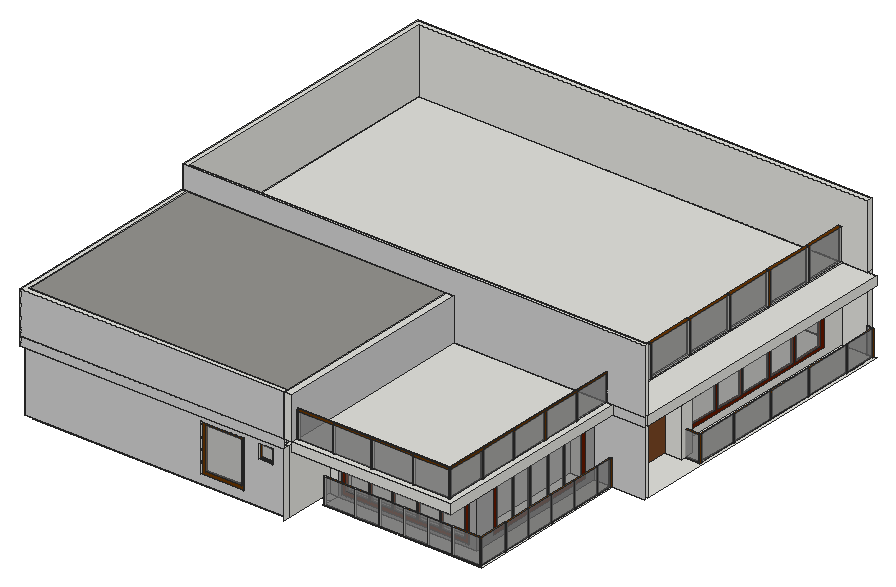
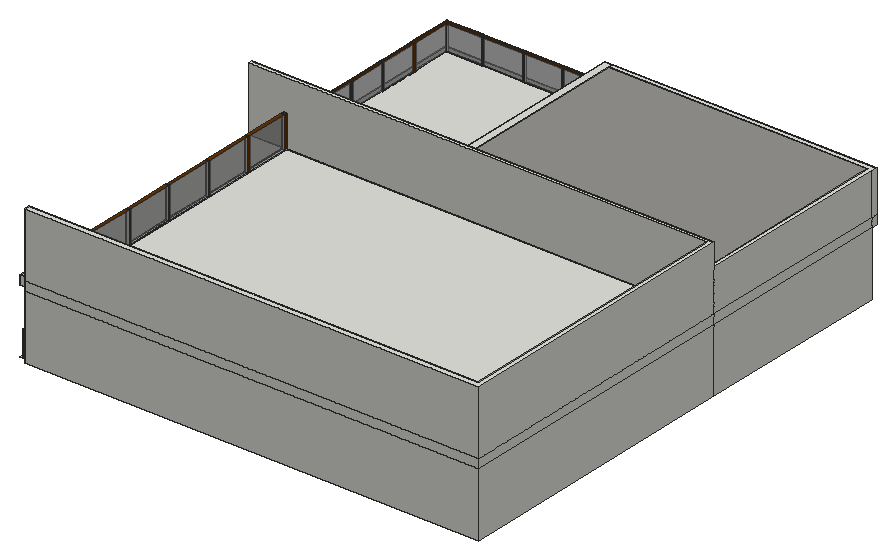
# SketchUp Ruby script. Lengths in inches.
U = 1.inch
M = Sketchup.active_model
def pt(a) = Geom::Point3d.new(a.map { |v| v * U })
def face(e, loops, mat)
  f = e.add_face(loops[0].map { |a| pt(a) })
  loops[1..].each { |l| e.add_face(l.map { |a| pt(a) }).erase! }
  f.material = f.back_material = mat if mat
  f
end
# faces: each face lists its corners as indices into pts; further lists are holes
def faces(e, pts, list, mat = nil) = list.each { |f| face(e, (f[0].is_a?(Array) ? f : [f]).map { |l| l.map { |i| pts[i] } }, mat) }
# xy, xz, yz: faces in a plane at the given z, y or x. An outline is a flat list of corners, or four numbers for a rectangle; further outlines are holes
def ring(l) = l.size == 4 ? [[l[0], l[1]], [l[2], l[1]], [l[2], l[3]], [l[0], l[3]]] : l.each_slice(2).to_a
def flat(e, list, mat, &to3) = list.each { |f| face(e, (f[0].is_a?(Array) ? f : [f]).map { |l| ring(l).map { |u, v| to3.(u, v) } }, mat) }
def xy(e, z, list, mat = nil) = flat(e, list, mat) { |x, y| [x, y, z] }
def xz(e, y, list, mat = nil) = flat(e, list, mat) { |x, z| [x, y, z] }
def yz(e, x, list, mat = nil) = flat(e, list, mat) { |y, z| [x, y, z] }
def lines(e, pts, list) = list.each { |a, b| e.add_line(pt(pts[a]), pt(pts[b])) }
# prism: a flat outline (further loops are holes) pulled along v
def prism(e, loops, v, mat = nil)
  f = face(e, loops, mat); d = Geom::Vector3d.new(v.map { |x| x * U })
  f.pushpull(f.normal.samedirection?(d) ? d.length : -d.length)
end
def box(e, o, s, mat = nil) = prism(e, [[o, [o[0] + s[0], o[1], o[2]], [o[0] + s[0], o[1] + s[1], o[2]], [o[0], o[1] + s[1], o[2]]]], [0, 0, s[2]], mat)
def at(x, y, z, deg = 0) = Geom::Transformation.translation(pt([x, y, z])) * Geom::Transformation.rotation(ORIGIN, Z_AXIS, deg.degrees)
def axes(o, x, y, z) = Geom::Transformation.new([*x, 0, *y, 0, *z, 0, *pt(o).to_a, 1])
def part(name) = M.definitions.add(name)
# library, detail: a bought-in or finely detailed component or shape, given as its bounding box
def library(name, o, s) = part(name).tap { |d| box(d.entities, o, s) }
def detail(e, o, s) = box(e.add_group.entities, o, s)
def put(e, d, t, mat = nil) = e.add_instance(d, t).tap { |i| i.material = mat if mat }
def group(e, t, mat = nil) = e.add_group.tap { |g| g.transformation = t; g.material = mat if mat }.entities
root = M.entities
M.materials.add("[Carrera Marble]").color = [207, 207, 207]
M.materials.add("[Color B08]").color = [102, 25, 0]
M.materials.add("[Color C08]").color = [102, 51, 0]
M.materials.add("[Granite Light Gray]").color = [149, 148, 144]
M.materials.add("[Stone Vein Gray]").color = [166, 165, 165]
M.materials.add("[Translucent Glass Gray]").color = [128, 128, 128]
M.materials["[Translucent Glass Gray]"].alpha = 0.5
M.materials.add("[Wood Veneer 01]").color = [120, 70, 37]
c1 = part("Group\#3")
xy(c1.entities,0,[[0,0,23.0625,440.625]],"[Color B08]")
xy(c1.entities,14.28,[[0,14.28,23.0625,92.65],[0,98.4,23.0625,173.71],[0,179.46,23.0625,261.65],[0,267.4,23.0625,340.59],[0,346.34,23.0625,426.35]],"[Color B08]")
xy(c1.entities,204.03,[[0,14.28,23.0625,92.65],[0,98.4,23.0625,173.71],[0,179.46,23.0625,261.65],[0,267.4,23.0625,340.59],[0,346.34,23.0625,426.35]],"[Color B08]")
xy(c1.entities,218.3125,[[0,0,23.0625,440.625]],"[Color B08]")
xz(c1.entities,0,[[0,0,23.0625,218.3125]],"[Color B08]")
xz(c1.entities,14.28,[[0,14.28,23.0625,204.03]],"[Color B08]")
xz(c1.entities,92.65,[[0,14.28,23.0625,204.03]],"[Color B08]")
xz(c1.entities,98.4,[[0,14.28,23.0625,204.03]],"[Color B08]")
xz(c1.entities,173.71,[[0,14.28,23.0625,204.03]],"[Color B08]")
xz(c1.entities,179.46,[[0,14.28,23.0625,204.03]],"[Color B08]")
xz(c1.entities,261.65,[[0,14.28,23.0625,204.03]],"[Color B08]")
xz(c1.entities,267.4,[[0,14.28,23.0625,204.03]],"[Color B08]")
xz(c1.entities,340.59,[[0,14.28,23.0625,204.03]],"[Color B08]")
xz(c1.entities,346.34,[[0,14.28,23.0625,204.03]],"[Color B08]")
xz(c1.entities,426.35,[[0,14.28,23.0625,204.03]],"[Color B08]")
xz(c1.entities,440.625,[[0,0,23.0625,218.3125]],"[Color B08]")
yz(c1.entities,0,[[[0,0,440.625,218.3125],[179.46,14.28,261.65,204.03],[346.34,14.28,426.35,204.03],[14.28,14.28,92.65,204.03],[98.4,14.28,173.71,204.03],[267.4,14.28,340.59,204.03]]],"[Color B08]")
yz(c1.entities,23.0625,[[[0,0,440.625,218.3125],[179.46,14.28,261.65,204.03],[346.34,14.28,426.35,204.03],[14.28,14.28,92.65,204.03],[98.4,14.28,173.71,204.03],[267.4,14.28,340.59,204.03]]],"[Color B08]")
yz(c1.entities,23.0625,[[14.28,14.28,92.65,204.03],[98.4,14.28,173.71,204.03],[179.46,14.28,261.65,204.03],[267.4,14.28,340.59,204.03],[346.34,14.28,426.35,204.03]],"[Translucent Glass Gray]")
c2 = part("Group\#1")
xy(c2.entities,0,[[0,0,21.625,260.4375]],"[Color C08]")
xy(c2.entities,20.42,[[0,20.42,21.625,240.02]],"[Color C08]")
xy(c2.entities,312.95,[[0,20.42,21.625,240.02]],"[Color C08]")
xy(c2.entities,333.375,[[0,0,21.625,260.4375]],"[Color C08]")
xz(c2.entities,0,[[0,0,21.625,333.375]],"[Color C08]")
xz(c2.entities,20.42,[[0,20.42,21.625,312.95]],"[Color C08]")
xz(c2.entities,240.02,[[0,20.42,21.625,312.95]],"[Color C08]")
xz(c2.entities,260.4375,[[0,0,21.625,333.375]],"[Color C08]")
yz(c2.entities,0,[[[0,0,260.4375,333.375],[20.42,20.42,240.02,312.95]]],"[Color C08]")
yz(c2.entities,21.625,[[[0,0,260.4375,333.375],[20.42,20.42,240.02,312.95]]],"[Color C08]")
yz(c2.entities,21.625,[[20.42,20.42,240.02,312.95]],"[Translucent Glass Gray]")
xy(root,960,[[9,213.0625,482.6875,573],[9,579,791.375,1111.6875]])
xy(root,966,[[0,207.0625,0,573,9,573,9,213.0625,482.6875,213.0625,482.6875,308.3125,607.75,308.3125,607.75,573,766.0625,573,766.0625,301.1875,491.3125,301.1875,491.3125,207.0625],[9,213.0625,482.6875,573],[506.0625,267.5625,801.71,267.5625,801.71,573,799.5,573,799.5,268.8125,506.0625,268.8125],[506.0625,268.8125,509.36,270.8125],[509.36,268.8125,564.18,270.8125],
  [564.18,268.8125,565.36,270.8125],[565.36,268.8125,609.49,270.8125],[609.49,268.8125,610.67,270.8125],[610.67,268.8125,654.81,270.8125],[654.81,268.8125,655.98,270.8125],
  [655.98,268.8125,700.12,270.8125],[700.12,268.8125,701.3,270.8125],[701.3,268.8125,745.43,270.8125],[745.43,268.8125,746.61,270.8125],[746.61,268.8125,797.5,270.8125],
  [797.5,268.8125,799.5,270.8125],[506.0625,270.8125,797.5,270.8125,797.5,573,766.0625,573,766.0625,301.1875,506.0625,301.1875],[797.5,270.8125,799.5,326.79],[491.3125,282.8125,506.0625,301.1875],[482.6875,308.3125,607.75,573],
  [797.5,326.79,799.5,327.91],[797.5,327.91,799.5,380.04],[797.5,380.04,799.5,381.16],[797.5,381.16,799.5,433.29],[797.5,433.29,799.5,434.41],
  [797.5,434.41,799.5,486.54],[797.5,486.54,799.5,487.66],[797.5,487.66,799.5,539.79],[797.5,539.79,799.5,540.91],[797.5,540.91,799.5,569.88],
  [797.5,569.88,799.5,573],[9,579,791.375,1111.6875],[797.375,579,861.375,579,861.375,1111.6875,797.375,1111.6875,797.375,723.02,828.5625,723.02,828.5625,710.0625,854.8125,710.0625,854.8125,1110.1875,845.0625,1110.1875,845.0625,1110.75,856.8125,1110.75,856.8125,706.6875,828.5625,706.6875,828.5625,699.0625,797.375,699.0625],[828.5625,706.6875,854.8125,710.0625],[854.8125,706.6875,856.8125,710.0625],
  [854.8125,710.0625,856.8125,784.92],[854.8125,784.92,856.8125,787.22],[854.8125,787.22,856.8125,872.67],[854.8125,872.67,856.8125,874.97],[854.8125,874.97,856.8125,960.42],
  [854.8125,960.42,856.8125,962.72],[854.8125,962.72,856.8125,1048.17],[854.8125,1048.17,856.8125,1050.47],[854.8125,1050.47,856.8125,1110.1875],[845.0625,1110.1875,854.8125,1110.75],
  [854.8125,1110.1875,856.8125,1110.75]])
xy(root,971.4,[[514.9,301.1875,750.72,321.75]])
xy(root,976.89,[[739.4375,339.98,766.0625,551.41]])
xy(root,976.93,[[791.375,750.16,797.375,1072.78]])
xy(root,981.52,[[327.22,207.0625,407.72,213.0625]])
xy(root,1014,[[506.0625,268.8125,509.36,270.8125],[509.36,268.8125,564.18,270.8125],[564.18,268.8125,565.36,270.8125],[565.36,268.8125,609.49,270.8125],[609.49,268.8125,610.67,270.8125],
  [610.67,268.8125,654.81,270.8125],[654.81,268.8125,655.98,270.8125],[655.98,268.8125,700.12,270.8125],[700.12,268.8125,701.3,270.8125],[701.3,268.8125,745.43,270.8125],
  [745.43,268.8125,746.61,270.8125],[746.61,268.8125,797.5,270.8125],[797.5,268.8125,799.5,270.8125],[797.5,270.8125,799.5,326.79],[797.5,326.79,799.5,327.91],
  [797.5,327.91,799.5,380.04],[797.5,380.04,799.5,381.16],[797.5,381.16,799.5,433.29],[797.5,433.29,799.5,434.41],[797.5,434.41,799.5,486.54],
  [797.5,486.54,799.5,487.66],[797.5,487.66,799.5,539.79],[797.5,539.79,799.5,540.91],[797.5,540.91,799.5,569.88],[797.5,569.88,799.5,573],
  [828.5625,706.6875,854.8125,710.0625],[854.8125,706.6875,856.8125,710.0625],[854.8125,710.0625,856.8125,784.92],[854.8125,784.92,856.8125,787.22],[854.8125,787.22,856.8125,872.67],
  [854.8125,872.67,856.8125,874.97],[854.8125,874.97,856.8125,960.42],[854.8125,960.42,856.8125,962.72],[854.8125,962.72,856.8125,1048.17],[854.8125,1048.17,856.8125,1050.47],
  [854.8125,1050.47,856.8125,1110.1875],[845.0625,1110.1875,854.8125,1110.75],[854.8125,1110.1875,856.8125,1110.75]],"[Color C08]")
xy(root,1044.6875,[[434.39,207.0625,461.57,213.0625]])
xy(root,1070.65,[[327.22,207.0625,407.72,213.0625]])
xy(root,1071.875,[[434.39,207.0625,461.57,213.0625]])
xy(root,1073.39,[[739.4375,339.98,766.0625,551.41]])
xy(root,1075.81,[[791.375,750.16,797.375,1072.78]])
xy(root,1078.15,[[514.9,301.1875,750.72,321.75]])
xy(root,1086,[[0,195.6875,491.3125,207.0625],[506.0625,195.6875,506.0625,301.1875,766.0625,301.1875,766.0625,573,801.71,573,801.71,195.6875],[0,207.0625,0,573,9,573,9,213.0625,482.6875,213.0625,482.6875,308.3125,607.75,308.3125,607.75,573,766.0625,573,766.0625,301.1875,491.3125,301.1875,491.3125,207.0625],[482.6875,308.3125,607.75,573],[797.375,579,861.375,699.0625],
  [797.375,699.0625,828.5625,723.02],[828.5625,699.0625,861.375,723.02],[797.375,723.02,861.375,1111.6875]])
xy(root,1098,[[9,579,791.375,1111.6875]])
xy(root,1103,[[0,195.6875,0,573,9,573,9,204.6875,491.3125,204.6875,491.3125,195.6875],[491.3125,195.6875,506.0625,573],[506.0625,195.6875,801.71,195.6875,801.71,573,791.02,573,791.02,206.3125,506.0625,206.3125],[9,204.6875,491.3125,573],[506.0625,206.3125,510.14,208.3125],
  [510.14,206.3125,572.71,208.3125],[572.71,206.3125,575.55,208.3125],[575.55,206.3125,644.96,208.3125],[644.96,206.3125,647.8,208.3125],[647.8,206.3125,721.78,208.3125],
  [721.78,206.3125,724.61,208.3125],[724.61,206.3125,789.02,208.3125],[789.02,206.3125,791.02,208.375],[506.0625,208.3125,789.02,573],[789.02,208.375,791.02,282.44],
  [789.02,282.44,791.02,285.25],[789.02,285.25,791.02,355.76],[789.02,355.76,791.02,358.5625],[789.02,358.5625,791.02,429.07],[789.02,429.07,791.02,431.875],
  [789.02,431.875,791.02,502.38],[789.02,502.38,791.02,505.1875],[789.02,505.1875,791.02,573],[9,579,791.375,1111.6875],[791.375,579,797.375,583.78],
  [797.375,579,861.375,1111.6875],[791.375,583.78,797.375,666.05],[791.375,666.05,797.375,668.89],[791.375,668.89,797.375,758.17],[791.375,758.17,797.375,761.01],
  [791.375,761.01,797.375,850.3],[791.375,850.3,797.375,853.14],[791.375,853.14,797.375,942.42],[791.375,942.42,797.375,945.26],[791.375,945.26,797.375,1034.55],
  [791.375,1034.55,797.375,1037.39],[791.375,1037.39,797.375,1111.6875]])
xy(root,1151,[[506.0625,206.3125,510.14,208.3125],[510.14,206.3125,572.71,208.3125],[572.71,206.3125,575.55,208.3125],[575.55,206.3125,644.96,208.3125],[644.96,206.3125,647.8,208.3125],
  [647.8,206.3125,721.78,208.3125],[721.78,206.3125,724.61,208.3125],[724.61,206.3125,789.02,208.3125],[789.02,206.3125,791.02,208.25],[789.02,208.25,791.02,208.375],
  [789.02,208.375,791.02,282.44],[789.02,282.44,791.02,285.25],[789.02,285.25,791.02,355.76],[789.02,355.76,791.02,358.5625],[789.02,358.5625,791.02,429.07],
  [789.02,429.07,791.02,431.875],[789.02,431.875,791.02,502.38],[789.02,502.38,791.02,505.1875],[789.02,505.1875,791.02,573]])
xy(root,1154.6875,[[789.02,208.25,791.02,208.3125]])
xy(root,1154.6875,[[506.0625,206.3125,789.02,208.3125],[789.02,206.3125,791.02,208.25],[789.02,208.3125,791.02,573]],"[Color C08]")
xy(root,1163,[[791.375,579,797.375,583.78],[791.375,583.78,797.375,666.05],[791.375,666.05,797.375,668.89],[791.375,668.89,797.375,758.17],[791.375,758.17,797.375,761.01],
  [791.375,761.01,797.375,850.3],[791.375,850.3,797.375,853.14],[791.375,853.14,797.375,942.42],[791.375,942.42,797.375,945.26],[791.375,945.26,797.375,1034.55],
  [791.375,1034.55,797.375,1037.39],[791.375,1037.39,797.375,1111.6875]],"[Color C08]")
xy(root,1173.9375,[[9,204.6875,491.3125,573]])
xy(root,1181.25,[[0,195.6875,491.3125,195.6875,491.3125,204.6875,9,204.6875,9,573,0,573],[491.3125,195.6875,506.0625,573]])
xy(root,1181.25,[[9,204.6875,491.3125,573]],"[Granite Light Gray]")
xy(root,1223,[[0,573,861.375,573,861.375,579,9,579,9,1111.6875,845.0625,1111.6875,845.0625,1120.6875,0,1120.6875]])
xz(root,195.6875,[[506.0625,1086,801.71,1103],[491.3125,1103,506.0625,1181.25]])
xz(root,195.6875,[[0,1086,491.3125,1103],[0,1103,491.3125,1181.25]],"[Carrera Marble]")
xz(root,204.6875,[[9,1103,491.3125,1173.9375],[9,1173.9375,491.3125,1181.25]])
xz(root,206.3125,[[506.0625,1103,510.14,1151],[572.71,1103,575.55,1151],[644.96,1103,647.8,1151],[721.78,1103,724.61,1151],[789.02,1103,791.02,1151],
  [506.0625,1151,510.14,1154.6875],[510.14,1151,572.71,1154.6875],[572.71,1151,575.55,1154.6875],[575.55,1151,644.96,1154.6875],[644.96,1151,647.8,1154.6875],
  [647.8,1151,721.78,1154.6875],[721.78,1151,724.61,1154.6875],[724.61,1151,789.02,1154.6875],[789.02,1151,791.02,1154.6875]],"[Color C08]")
xz(root,206.3125,[[510.14,1103,572.71,1151],[575.55,1103,644.96,1151],[647.8,1103,721.78,1151],[724.61,1103,789.02,1151]],"[Translucent Glass Gray]")
xz(root,207.0625,[[[0,966,491.3125,1086],[327.22,981.52,407.72,1070.65],[434.39,1044.6875,461.57,1071.875]]],"[Carrera Marble]")
xz(root,208.25,[[789.02,1151,791.02,1154.6875]])
xz(root,208.3125,[[506.0625,1103,510.14,1151],[572.71,1103,575.55,1151],[644.96,1103,647.8,1151],[721.78,1103,724.61,1151],[506.0625,1151,789.02,1154.6875]],"[Color C08]")
xz(root,208.3125,[[510.14,1103,572.71,1151],[575.55,1103,644.96,1151],[647.8,1103,721.78,1151],[724.61,1103,789.02,1151]],"[Translucent Glass Gray]")
xz(root,213.0625,[[9,960,482.6875,966],[[9,966,482.6875,1086],[327.22,981.52,407.72,1070.65],[434.39,1044.6875,461.57,1071.875]],[9,1086,482.6875,1097]])
xz(root,268.8125,[[506.0625,966,509.36,1014],[564.18,966,565.36,1014],[609.49,966,610.67,1014],[654.81,966,655.98,1014],[700.12,966,701.3,1014],
  [745.43,966,746.61,1014],[797.5,966,799.5,1014]],"[Color C08]")
xz(root,268.8125,[[509.36,966,564.18,1014],[565.36,966,609.49,1014],[610.67,966,654.81,1014],[655.98,966,700.12,1014],[701.3,966,745.43,1014],
  [746.61,966,797.5,1014]],"[Translucent Glass Gray]")
xz(root,270.8125,[[564.18,966,565.36,1014],[609.49,966,610.67,1014],[654.81,966,655.98,1014],[700.12,966,701.3,1014],[745.43,966,746.61,1014],
  [797.5,966,799.5,1014]])
xz(root,270.8125,[[509.36,966,564.18,1014],[565.36,966,609.49,1014],[610.67,966,654.81,1014],[655.98,966,700.12,1014],[701.3,966,745.43,1014],
  [746.61,966,797.5,1014]],"[Translucent Glass Gray]")
xz(root,282.44,[[789.02,1103,791.02,1151]])
xz(root,285.25,[[789.02,1103,791.02,1151]])
xz(root,301.1875,[[491.3125,966,506.0625,1086]])
xz(root,301.1875,[[[506.0625,966,766.0625,1086],[514.9,971.4,750.72,1078.15]]],"[Stone Vein Gray]")
xz(root,321.75,[[514.9,971.4,750.72,1078.15]])
xz(root,326.79,[[797.5,966,799.5,1014]])
xz(root,327.91,[[797.5,966,799.5,1014]])
xz(root,339.98,[[739.4375,976.89,766.0625,1073.39]])
xz(root,355.76,[[789.02,1103,791.02,1151]])
xz(root,358.5625,[[789.02,1103,791.02,1151]])
xz(root,380.04,[[797.5,966,799.5,1014]])
xz(root,381.16,[[797.5,966,799.5,1014]])
xz(root,429.07,[[789.02,1103,791.02,1151]])
xz(root,431.875,[[789.02,1103,791.02,1151]])
xz(root,433.29,[[797.5,966,799.5,1014]])
xz(root,434.41,[[797.5,966,799.5,1014]])
xz(root,486.54,[[797.5,966,799.5,1014]])
xz(root,487.66,[[797.5,966,799.5,1014]])
xz(root,502.38,[[789.02,1103,791.02,1151]])
xz(root,505.1875,[[789.02,1103,791.02,1151]])
xz(root,539.79,[[797.5,966,799.5,1014]])
xz(root,540.91,[[797.5,966,799.5,1014]])
xz(root,551.41,[[739.4375,976.89,766.0625,1073.39]])
xz(root,569.88,[[797.5,966,799.5,1014]])
xz(root,573,[[9,960,482.6875,966],[0,966,9,1086],[9,966,482.6875,1086],[482.6875,966,607.75,1086],[607.75,966,766.0625,1086],
  [797.5,966,799.5,1014],[0,1086,9,1103],[9,1086,482.6875,1097],[482.6875,1086,613.75,1103],[613.75,1086,801.71,1103],
  [9,1097,482.6875,1103],[0,1103,9,1181.25],[9,1103,491.3125,1173.9375],[491.3125,1103,506.0625,1181.25],[789.02,1103,791.02,1151],
  [789.02,1151,791.02,1154.6875],[9,1173.9375,491.3125,1181.25]])
xz(root,573,[[766.0625,966,797.5,966,797.5,1014,799.5,1014,799.5,966,861.375,966,861.375,1086,766.0625,1086],[801.71,1086,861.375,1103],[506.0625,1103,789.02,1103,789.02,1154.6875,791.02,1154.6875,791.02,1103,861.375,1103,861.375,1223,0,1223,0,1181.25,506.0625,1181.25]],"[Carrera Marble]")
xz(root,579,[[9,960,791.375,966],[9,966,791.375,1086],[797.375,966,861.375,1086],[9,1086,791.375,1098],[797.375,1086,861.375,1103],
  [9,1098,791.375,1103],[9,1103,9,1223,861.375,1223,861.375,1103,797.375,1103,797.375,1163,791.375,1163,791.375,1103]])
xz(root,579,[[791.375,1103,797.375,1163]],"[Color C08]")
xz(root,583.78,[[791.375,1103,797.375,1163]])
xz(root,666.05,[[791.375,1103,797.375,1163]])
xz(root,668.89,[[791.375,1103,797.375,1163]])
xz(root,699.0625,[[797.375,966,828.5625,1086]])
xz(root,706.6875,[[854.8125,966,856.8125,1014]],"[Color C08]")
xz(root,706.6875,[[828.5625,966,854.8125,1014]],"[Translucent Glass Gray]")
xz(root,710.0625,[[854.8125,966,856.8125,1014]])
xz(root,710.0625,[[828.5625,966,854.8125,1014]],"[Translucent Glass Gray]")
xz(root,723.02,[[797.375,966,828.5625,1086]])
xz(root,750.16,[[791.375,976.93,797.375,1075.81]])
xz(root,758.17,[[791.375,1103,797.375,1163]])
xz(root,761.01,[[791.375,1103,797.375,1163]])
xz(root,784.92,[[854.8125,966,856.8125,1014]])
xz(root,787.22,[[854.8125,966,856.8125,1014]])
xz(root,850.3,[[791.375,1103,797.375,1163]])
xz(root,853.14,[[791.375,1103,797.375,1163]])
xz(root,872.67,[[854.8125,966,856.8125,1014]])
xz(root,874.97,[[854.8125,966,856.8125,1014]])
xz(root,942.42,[[791.375,1103,797.375,1163]])
xz(root,945.26,[[791.375,1103,797.375,1163]])
xz(root,960.42,[[854.8125,966,856.8125,1014]])
xz(root,962.72,[[854.8125,966,856.8125,1014]])
xz(root,1034.55,[[791.375,1103,797.375,1163]])
xz(root,1037.39,[[791.375,1103,797.375,1163]])
xz(root,1048.17,[[854.8125,966,856.8125,1014]])
xz(root,1050.47,[[854.8125,966,856.8125,1014]])
xz(root,1072.78,[[791.375,976.93,797.375,1075.81]])
xz(root,1110.1875,[[845.0625,966,854.8125,1014]],"[Translucent Glass Gray]")
xz(root,1110.75,[[845.0625,966,854.8125,1014]])
xz(root,1110.75,[[854.8125,966,856.8125,1014]],"[Color C08]")
xz(root,1111.6875,[[9,960,791.375,966],[9,966,791.375,1086],[797.375,966,845.0625,1086],[9,1086,791.375,1098],[797.375,1086,845.0625,1103],
  [845.0625,1086,861.375,1103],[9,1098,791.375,1103],[9,1103,791.375,1103,791.375,1163,797.375,1163,797.375,1103,845.0625,1103,845.0625,1223,9,1223],[791.375,1103,797.375,1163]])
xz(root,1120.6875,[[0,966,845.0625,1086],[0,1086,845.0625,1103],[0,1103,845.0625,1223]])
yz(root,0,[[207.0625,966,573,1086],[573,966,1120.6875,1086],[195.6875,1086,207.0625,1103],[207.0625,1086,573,1103],[573,1086,1120.6875,1103],
  [195.6875,1103,207.0625,1181.25],[207.0625,1103,573,1181.25],[573,1103,1120.6875,1223]])
yz(root,9,[[213.0625,960,222,966],[222,960,573,966],[579,960,1111.6875,966],[213.0625,966,222,1086],[222,966,573,1086],
  [579,966,1111.6875,1086],[213.0625,1086,222,1097],[222,1086,573,1097],[579,1086,1111.6875,1098],[213.0625,1097,222,1103],
  [222,1097,573,1103],[579,1098,613.53,1103],[613.53,1098,667.72,1103],[667.72,1098,1111.6875,1103],[204.6875,1103,213.0625,1173.9375],
  [213.0625,1103,222,1173.9375],[222,1103,573,1173.9375],[579,1103,1111.6875,1223],[204.6875,1173.9375,213.0625,1181.25],[213.0625,1173.9375,222,1181.25],
  [222,1173.9375,573,1181.25]])
yz(root,327.22,[[207.0625,981.52,213.0625,1070.65]])
yz(root,407.72,[[207.0625,981.52,213.0625,1070.65]])
yz(root,434.39,[[207.0625,1044.6875,213.0625,1071.875]])
yz(root,461.57,[[207.0625,1044.6875,213.0625,1071.875]])
yz(root,482.6875,[[213.0625,960,308.3125,966],[308.3125,960,433.03,966],[433.03,960,458.59,966],[458.59,960,573,966],[213.0625,966,573,1086],
  [213.0625,1086,573,1097]])
yz(root,491.3125,[[195.6875,966,207.0625,1086],[207.0625,966,301.1875,1086],[195.6875,1103,204.6875,1181.25],[204.6875,1103,573,1173.9375],[204.6875,1173.9375,573,1181.25]])
yz(root,506.0625,[[268.8125,966,270.8125,1014],[206.3125,1103,208.3125,1151],[206.3125,1151,208.3125,1154.6875]])
yz(root,506.0625,[[195.6875,1103,206.3125,1103,206.3125,1154.6875,208.3125,1154.6875,208.3125,1103,573,1103,573,1181.25,195.6875,1181.25]],"[Carrera Marble]")
yz(root,509.36,[[268.8125,966,270.8125,1014]])
yz(root,510.14,[[206.3125,1103,208.3125,1151]])
yz(root,514.9,[[301.1875,971.4,321.75,1078.15]])
yz(root,564.18,[[268.8125,966,270.8125,1014]])
yz(root,565.36,[[268.8125,966,270.8125,1014]])
yz(root,572.71,[[206.3125,1103,208.3125,1151]])
yz(root,575.55,[[206.3125,1103,208.3125,1151]])
yz(root,609.49,[[268.8125,966,270.8125,1014]])
yz(root,610.67,[[268.8125,966,270.8125,1014]])
yz(root,644.96,[[206.3125,1103,208.3125,1151]])
yz(root,647.8,[[206.3125,1103,208.3125,1151]])
yz(root,654.81,[[268.8125,966,270.8125,1014]])
yz(root,655.98,[[268.8125,966,270.8125,1014]])
yz(root,700.12,[[268.8125,966,270.8125,1014]])
yz(root,701.3,[[268.8125,966,270.8125,1014]])
yz(root,721.78,[[206.3125,1103,208.3125,1151]])
yz(root,724.61,[[206.3125,1103,208.3125,1151]])
yz(root,739.4375,[[339.98,976.89,551.41,1073.39]])
yz(root,745.43,[[268.8125,966,270.8125,1014]])
yz(root,746.61,[[268.8125,966,270.8125,1014]])
yz(root,750.72,[[301.1875,971.4,321.75,1078.15]])
yz(root,766.0625,[[[301.1875,966,573,1086],[339.98,976.89,551.41,1073.39]]],"[Stone Vein Gray]")
yz(root,789.02,[[206.3125,1103,208.3125,1151],[208.3125,1103,208.375,1151],[206.3125,1151,208.25,1154.6875]])
yz(root,789.02,[[282.44,1103,285.25,1151],[355.76,1103,358.5625,1151],[429.07,1103,431.875,1151],[502.38,1103,505.1875,1151],[208.3125,1151,573,1154.6875]],"[Color C08]")
yz(root,789.02,[[208.375,1103,282.44,1151],[285.25,1103,355.76,1151],[358.5625,1103,429.07,1151],[431.875,1103,502.38,1151],[505.1875,1103,573,1151]],"[Translucent Glass Gray]")
yz(root,791.02,[[208.3125,1103,208.375,1151],[208.25,1151,208.3125,1154.6875]])
yz(root,791.02,[[206.3125,1103,208.3125,1151],[282.44,1103,285.25,1151],[355.76,1103,358.5625,1151],[429.07,1103,431.875,1151],[502.38,1103,505.1875,1151],
  [206.3125,1151,208.25,1154.6875],[208.3125,1151,282.44,1154.6875],[282.44,1151,285.25,1154.6875],[285.25,1151,355.76,1154.6875],[355.76,1151,358.5625,1154.6875],
  [358.5625,1151,429.07,1154.6875],[429.07,1151,431.875,1154.6875],[431.875,1151,502.38,1154.6875],[502.38,1151,505.1875,1154.6875],[505.1875,1151,573,1154.6875]],"[Color C08]")
yz(root,791.02,[[208.375,1103,282.44,1151],[285.25,1103,355.76,1151],[358.5625,1103,429.07,1151],[431.875,1103,502.38,1151],[505.1875,1103,573,1151]],"[Translucent Glass Gray]")
yz(root,791.375,[[579,960,1050.06,966],[1050.06,960,1060.81,966],[1060.81,960,1111.6875,966],[[579,966,1111.6875,1086],[750.16,976.93,1072.78,1075.81]],[579,1086,1111.6875,1098],
  [579,1098,1111.6875,1103]])
yz(root,791.375,[[666.05,1103,668.89,1163],[758.17,1103,761.01,1163],[850.3,1103,853.14,1163],[942.42,1103,945.26,1163],[1034.55,1103,1037.39,1163]],"[Color C08]")
yz(root,791.375,[[583.78,1103,666.05,1163],[668.89,1103,758.17,1163],[761.01,1103,850.3,1163],[853.14,1103,942.42,1163],[945.26,1103,1034.55,1163],
  [1037.39,1103,1111.6875,1163]],"[Translucent Glass Gray]")
yz(root,797.375,[[[723.02,966,1111.6875,1086],[750.16,976.93,1072.78,1075.81]],[579,1086,1111.6875,1103]])
yz(root,797.375,[[579,1103,583.78,1163],[666.05,1103,668.89,1163],[758.17,1103,761.01,1163],[850.3,1103,853.14,1163],[942.42,1103,945.26,1163],
  [1034.55,1103,1037.39,1163]],"[Color C08]")
yz(root,797.375,[[583.78,1103,666.05,1163],[668.89,1103,758.17,1163],[761.01,1103,850.3,1163],[853.14,1103,942.42,1163],[945.26,1103,1034.55,1163],
  [1037.39,1103,1111.6875,1163]],"[Translucent Glass Gray]")
yz(root,797.375,[[579,966,699.0625,1086]],"[Wood Veneer 01]")
yz(root,797.5,[[268.8125,966,270.8125,1014]])
yz(root,797.5,[[326.79,966,327.91,1014],[380.04,966,381.16,1014],[433.29,966,434.41,1014],[486.54,966,487.66,1014],[539.79,966,540.91,1014],
  [569.88,966,573,1014]],"[Color C08]")
yz(root,797.5,[[270.8125,966,326.79,1014],[327.91,966,380.04,1014],[381.16,966,433.29,1014],[434.41,966,486.54,1014],[487.66,966,539.79,1014],
  [540.91,966,569.88,1014]],"[Translucent Glass Gray]")
yz(root,799.5,[[268.8125,966,270.8125,1014],[326.79,966,327.91,1014],[380.04,966,381.16,1014],[433.29,966,434.41,1014],[486.54,966,487.66,1014],
  [539.79,966,540.91,1014],[569.88,966,573,1014]],"[Color C08]")
yz(root,799.5,[[270.8125,966,326.79,1014],[327.91,966,380.04,1014],[381.16,966,433.29,1014],[434.41,966,486.54,1014],[487.66,966,539.79,1014],
  [540.91,966,569.88,1014]],"[Translucent Glass Gray]")
yz(root,801.71,[[195.6875,1086,573,1103]])
yz(root,828.5625,[[699.0625,966,706.6875,966,706.6875,1014,710.0625,1014,710.0625,966,723.02,966,723.02,1086,699.0625,1086],[706.6875,966,710.0625,1014]])
yz(root,845.0625,[[1110.1875,966,1110.75,1014],[1111.6875,966,1120.6875,1086],[1111.6875,1086,1120.6875,1103],[1111.6875,1103,1120.6875,1223]])
yz(root,854.8125,[[706.6875,966,710.0625,1014],[1048.17,966,1050.47,1014],[1110.1875,966,1110.75,1014]])
yz(root,854.8125,[[784.92,966,787.22,1014],[872.67,966,874.97,1014],[960.42,966,962.72,1014]],"[Color C08]")
yz(root,854.8125,[[710.0625,966,784.92,1014],[787.22,966,872.67,1014],[874.97,966,960.42,1014],[962.72,966,1048.17,1014],[1050.47,966,1110.1875,1014]],"[Translucent Glass Gray]")
yz(root,856.8125,[[706.6875,966,710.0625,1014],[784.92,966,787.22,1014],[872.67,966,874.97,1014],[960.42,966,962.72,1014],[1048.17,966,1050.47,1014],
  [1110.1875,966,1110.75,1014]],"[Color C08]")
yz(root,856.8125,[[710.0625,966,784.92,1014],[787.22,966,872.67,1014],[874.97,966,960.42,1014],[962.72,966,1048.17,1014],[1050.47,966,1110.1875,1014]],"[Translucent Glass Gray]")
yz(root,861.375,[[579,1086,1111.6875,1103]])
p = [[799.5,646.29,1014],[799.5,647.41,1014],[482.6875,553.77,1103],[482.6875,553.77,1097],[482.6875,213.0625,1103],[482.6875,213.0625,1097]]
lines(root,p,[[0,1],[2,3],[4,5]])
put(root,c1,axes([514.9,303.92,972.09],[0,-0.11844,0],[0.53518,0,0],[0,0,0.48898]))
put(root,c1,axes([763.93,339.98,976.89],[0.09257,0,0],[0,0.47986,0],[0,0,0.44203]))
put(root,c1,axes([792.53,750.55,976.93],[0.21,0,0],[0,0.7313,0],[0,0,0.45291]))
put(root,c2,axes([327.22,213.12,981.52],[0,-0.1652,0],[0.3091,0,0],[0,0,0.26597]))
put(root,c2,axes([434.39,209.34,1044.6875],[0,0.11448,0],[0.10439,0,0],[0,0,0.08155]))
